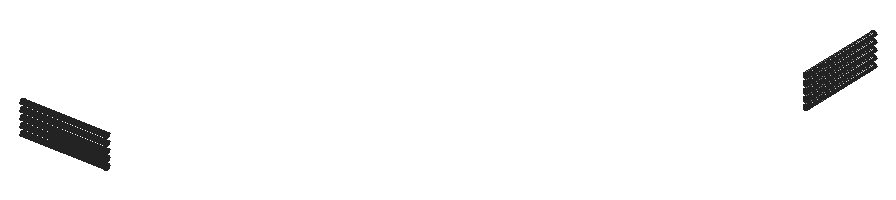
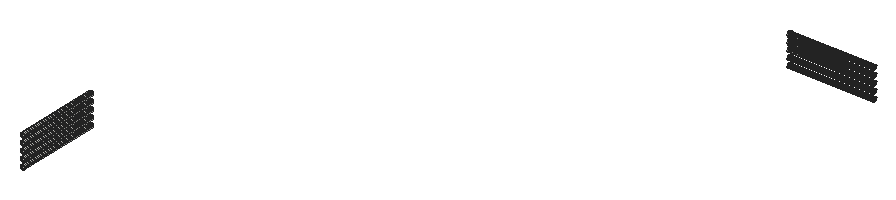
# SketchUp Ruby script. Lengths in inches.
U = 1.inch
M = Sketchup.active_model
def pt(a) = Geom::Point3d.new(a.map { |v| v * U })
def face(e, loops, mat)
  f = e.add_face(loops[0].map { |a| pt(a) })
  loops[1..].each { |l| e.add_face(l.map { |a| pt(a) }).erase! }
  f.material = f.back_material = mat if mat
  f
end
# faces: each face lists its corners as indices into pts; further lists are holes
def faces(e, pts, list, mat = nil) = list.each { |f| face(e, (f[0].is_a?(Array) ? f : [f]).map { |l| l.map { |i| pts[i] } }, mat) }
# xy, xz, yz: faces in a plane at the given z, y or x. An outline is a flat list of corners, or four numbers for a rectangle; further outlines are holes
def ring(l) = l.size == 4 ? [[l[0], l[1]], [l[2], l[1]], [l[2], l[3]], [l[0], l[3]]] : l.each_slice(2).to_a
def flat(e, list, mat, &to3) = list.each { |f| face(e, (f[0].is_a?(Array) ? f : [f]).map { |l| ring(l).map { |u, v| to3.(u, v) } }, mat) }
def xy(e, z, list, mat = nil) = flat(e, list, mat) { |x, y| [x, y, z] }
def xz(e, y, list, mat = nil) = flat(e, list, mat) { |x, z| [x, y, z] }
def yz(e, x, list, mat = nil) = flat(e, list, mat) { |y, z| [x, y, z] }
def lines(e, pts, list) = list.each { |a, b| e.add_line(pt(pts[a]), pt(pts[b])) }
# prism: a flat outline (further loops are holes) pulled along v
def prism(e, loops, v, mat = nil)
  f = face(e, loops, mat); d = Geom::Vector3d.new(v.map { |x| x * U })
  f.pushpull(f.normal.samedirection?(d) ? d.length : -d.length)
end
def box(e, o, s, mat = nil) = prism(e, [[o, [o[0] + s[0], o[1], o[2]], [o[0] + s[0], o[1] + s[1], o[2]], [o[0], o[1] + s[1], o[2]]]], [0, 0, s[2]], mat)
def at(x, y, z, deg = 0) = Geom::Transformation.translation(pt([x, y, z])) * Geom::Transformation.rotation(ORIGIN, Z_AXIS, deg.degrees)
def axes(o, x, y, z) = Geom::Transformation.new([*x, 0, *y, 0, *z, 0, *pt(o).to_a, 1])
def part(name) = M.definitions.add(name)
# library, detail: a bought-in or finely detailed component or shape, given as its bounding box
def library(name, o, s) = part(name).tap { |d| box(d.entities, o, s) }
def detail(e, o, s) = box(e.add_group.entities, o, s)
def put(e, d, t, mat = nil) = e.add_instance(d, t).tap { |i| i.material = mat if mat }
def group(e, t, mat = nil) = e.add_group.tap { |g| g.transformation = t; g.material = mat if mat }.entities
root = M.entities
p = [[922.01,48.34,1317.02],[922.01,47.38,1317.14],[778.64,47.38,1317.14],[778.64,48.34,1317.02],[922.01,49.29,1317.14],[778.64,49.29,1317.14],
  [1535.52,886.83,1317.14],[1536.47,886.83,1317.02],[1536.47,743.45,1317.02],[1535.52,743.45,1317.14],[1537.43,886.83,1317.14],[1537.43,743.45,1317.14],
  [922.01,46.5,1317.51],[778.64,46.5,1317.51],[922.01,50.18,1317.51],[778.64,50.18,1317.51],[1534.63,886.83,1317.51],[1534.63,743.45,1317.51],
  [1538.32,886.83,1317.51],[1538.32,743.45,1317.51],[922.01,45.73,1318.1],[778.64,45.73,1318.1],[922.01,50.95,1318.1],[778.64,50.95,1318.1],
  [1533.87,886.83,1318.1],[1533.87,743.45,1318.1],[1539.08,886.83,1318.1],[1539.08,743.45,1318.1],[922.01,45.15,1318.86],[778.64,45.15,1318.86],
  [922.01,51.53,1318.86],[778.64,51.53,1318.86],[1533.28,886.83,1318.86],[1533.28,743.45,1318.86],[1539.67,886.83,1318.86],[1539.67,743.45,1318.86],
  [922.01,44.78,1319.75],[778.64,44.78,1319.75],[922.01,51.9,1319.75],[778.64,51.9,1319.75],[1532.91,886.83,1319.75],[1532.91,743.45,1319.75],
  [1540.03,886.83,1319.75],[1540.03,743.45,1319.75],[922.01,44.65,1320.7],[778.64,44.65,1320.7],[922.01,52.03,1320.7],[778.64,52.03,1320.7],
  [1532.79,886.83,1320.7],[1532.79,743.45,1320.7],[1540.16,886.83,1320.7],[1540.16,743.45,1320.7],[922.01,44.78,1321.66],[778.64,44.78,1321.66],
  [922.01,51.9,1321.66],[778.64,51.9,1321.66],[1532.91,886.83,1321.66],[1532.91,743.45,1321.66],[1540.03,886.83,1321.66],[1540.03,743.45,1321.66],
  [922.01,45.15,1322.55],[778.64,45.15,1322.55],[922.01,51.53,1322.55],[778.64,51.53,1322.55],[1533.28,886.83,1322.55],[1533.28,743.45,1322.55],
  [1539.67,886.83,1322.55],[1539.67,743.45,1322.55],[922.01,45.73,1323.3125],[778.64,45.73,1323.3125],[922.01,50.95,1323.3125],[778.64,50.95,1323.3125],
  [1533.87,886.83,1323.3125],[1533.87,743.45,1323.3125],[1539.08,886.83,1323.3125],[1539.08,743.45,1323.3125],[922.01,46.5,1323.9],[778.64,46.5,1323.9],
  [922.01,50.18,1323.9],[778.64,50.18,1323.9],[1534.63,886.83,1323.9],[1534.63,743.45,1323.9],[1538.32,886.83,1323.9],[1538.32,743.45,1323.9],
  [922.01,47.38,1324.27],[778.64,47.38,1324.27],[922.01,49.29,1324.27],[778.64,49.29,1324.27],[1535.52,886.83,1324.27],[1535.52,743.45,1324.27],
  [1537.43,886.83,1324.27],[1537.43,743.45,1324.27],[922.01,48.34,1324.39],[778.64,48.34,1324.39],[1536.47,886.83,1324.39],[1536.47,743.45,1324.39],
  [922.01,48.34,1329.02],[922.01,47.38,1329.14],[778.64,47.38,1329.14],[778.64,48.34,1329.02],[922.01,49.29,1329.14],[778.64,49.29,1329.14],
  [1535.52,886.83,1329.14],[1536.47,886.83,1329.02],[1536.47,743.45,1329.02],[1535.52,743.45,1329.14],[1537.43,886.83,1329.14],[1537.43,743.45,1329.14],
  [922.01,46.5,1329.51],[778.64,46.5,1329.51],[922.01,50.18,1329.51],[778.64,50.18,1329.51],[1534.63,886.83,1329.51],[1534.63,743.45,1329.51],
  [1538.32,886.83,1329.51],[1538.32,743.45,1329.51],[922.01,45.73,1330.1],[778.64,45.73,1330.1],[922.01,50.95,1330.1],[778.64,50.95,1330.1],
  [1533.87,886.83,1330.1],[1533.87,743.45,1330.1],[1539.08,886.83,1330.1],[1539.08,743.45,1330.1],[922.01,45.15,1330.86],[778.64,45.15,1330.86],
  [922.01,51.53,1330.86],[778.64,51.53,1330.86],[1533.28,886.83,1330.86],[1533.28,743.45,1330.86],[1539.67,886.83,1330.86],[1539.67,743.45,1330.86],
  [922.01,44.78,1331.75],[778.64,44.78,1331.75],[922.01,51.9,1331.75],[778.64,51.9,1331.75],[1532.91,886.83,1331.75],[1532.91,743.45,1331.75],
  [1540.03,886.83,1331.75],[1540.03,743.45,1331.75],[922.01,44.65,1332.7],[778.64,44.65,1332.7],[922.01,52.03,1332.7],[778.64,52.03,1332.7],
  [1532.79,886.83,1332.7],[1532.79,743.45,1332.7],[1540.16,886.83,1332.7],[1540.16,743.45,1332.7],[922.01,44.78,1333.66],[778.64,44.78,1333.66],
  [922.01,51.9,1333.66],[778.64,51.9,1333.66],[1532.91,886.83,1333.66],[1532.91,743.45,1333.66],[1540.03,886.83,1333.66],[1540.03,743.45,1333.66],
  [922.01,45.15,1334.55],[778.64,45.15,1334.55],[922.01,51.53,1334.55],[778.64,51.53,1334.55],[1533.28,886.83,1334.55],[1533.28,743.45,1334.55],
  [1539.67,886.83,1334.55],[1539.67,743.45,1334.55],[922.01,45.73,1335.3125],[778.64,45.73,1335.3125],[922.01,50.95,1335.3125],[778.64,50.95,1335.3125],
  [1533.87,886.83,1335.3125],[1533.87,743.45,1335.3125],[1539.08,886.83,1335.3125],[1539.08,743.45,1335.3125],[922.01,46.5,1335.9],[778.64,46.5,1335.9],
  [922.01,50.18,1335.9],[778.64,50.18,1335.9],[1534.63,886.83,1335.9],[1534.63,743.45,1335.9],[1538.32,886.83,1335.9],[1538.32,743.45,1335.9],
  [922.01,47.38,1336.27],[778.64,47.38,1336.27],[922.01,49.29,1336.27],[778.64,49.29,1336.27],[1535.52,886.83,1336.27],[1535.52,743.45,1336.27],
  [1537.43,886.83,1336.27],[1537.43,743.45,1336.27],[922.01,48.34,1336.39],[778.64,48.34,1336.39],[1536.47,886.83,1336.39],[1536.47,743.45,1336.39],
  [922.01,48.34,1341.02],[922.01,47.38,1341.14],[778.64,47.38,1341.14],[778.64,48.34,1341.02],[922.01,49.29,1341.14],[778.64,49.29,1341.14],
  [1535.52,886.83,1341.14],[1536.47,886.83,1341.02],[1536.47,743.45,1341.02],[1535.52,743.45,1341.14],[1537.43,886.83,1341.14],[1537.43,743.45,1341.14],
  [922.01,46.5,1341.51],[778.64,46.5,1341.51],[922.01,50.18,1341.51],[778.64,50.18,1341.51],[1534.63,886.83,1341.51],[1534.63,743.45,1341.51],
  [1538.32,886.83,1341.51],[1538.32,743.45,1341.51],[922.01,45.73,1342.1],[778.64,45.73,1342.1],[922.01,50.95,1342.1],[778.64,50.95,1342.1],
  [1533.87,886.83,1342.1],[1533.87,743.45,1342.1],[1539.08,886.83,1342.1],[1539.08,743.45,1342.1],[922.01,45.15,1342.86],[778.64,45.15,1342.86],
  [922.01,51.53,1342.86],[778.64,51.53,1342.86],[1533.28,886.83,1342.86],[1533.28,743.45,1342.86],[1539.67,886.83,1342.86],[1539.67,743.45,1342.86],
  [922.01,44.78,1343.75],[778.64,44.78,1343.75],[922.01,51.9,1343.75],[778.64,51.9,1343.75],[1532.91,886.83,1343.75],[1532.91,743.45,1343.75],
  [1540.03,886.83,1343.75],[1540.03,743.45,1343.75],[922.01,44.65,1344.7],[778.64,44.65,1344.7],[922.01,52.03,1344.7],[778.64,52.03,1344.7],
  [1532.79,886.83,1344.7],[1532.79,743.45,1344.7],[1540.16,886.83,1344.7],[1540.16,743.45,1344.7],[922.01,44.78,1345.66],[778.64,44.78,1345.66],
  [922.01,51.9,1345.66],[778.64,51.9,1345.66],[1532.91,886.83,1345.66],[1532.91,743.45,1345.66],[1540.03,886.83,1345.66],[1540.03,743.45,1345.66],
  [922.01,45.15,1346.55],[778.64,45.15,1346.55],[922.01,51.53,1346.55],[778.64,51.53,1346.55],[1533.28,886.83,1346.55],[1533.28,743.45,1346.55],
  [1539.67,886.83,1346.55],[1539.67,743.45,1346.55],[922.01,45.73,1347.3125],[778.64,45.73,1347.3125],[922.01,50.95,1347.3125],[778.64,50.95,1347.3125],
  [1533.87,886.83,1347.3125],[1533.87,743.45,1347.3125],[1539.08,886.83,1347.3125],[1539.08,743.45,1347.3125],[922.01,46.5,1347.9],[778.64,46.5,1347.9],
  [922.01,50.18,1347.9],[778.64,50.18,1347.9],[1534.63,886.83,1347.9],[1534.63,743.45,1347.9],[1538.32,886.83,1347.9],[1538.32,743.45,1347.9],
  [922.01,47.38,1348.27],[778.64,47.38,1348.27],[922.01,49.29,1348.27],[778.64,49.29,1348.27],[1535.52,886.83,1348.27],[1535.52,743.45,1348.27],
  [1537.43,886.83,1348.27],[1537.43,743.45,1348.27],[922.01,48.34,1348.39],[778.64,48.34,1348.39],[1536.47,886.83,1348.39],[1536.47,743.45,1348.39],
  [922.01,48.34,1353.02],[922.01,47.38,1353.14],[778.64,47.38,1353.14],[778.64,48.34,1353.02],[922.01,49.29,1353.14],[778.64,49.29,1353.14],
  [1535.52,886.83,1353.14],[1536.47,886.83,1353.02],[1536.47,743.45,1353.02],[1535.52,743.45,1353.14],[1537.43,886.83,1353.14],[1537.43,743.45,1353.14],
  [922.01,46.5,1353.51],[778.64,46.5,1353.51],[922.01,50.18,1353.51],[778.64,50.18,1353.51],[1534.63,886.83,1353.51],[1534.63,743.45,1353.51],
  [1538.32,886.83,1353.51],[1538.32,743.45,1353.51],[922.01,45.73,1354.1],[778.64,45.73,1354.1],[922.01,50.95,1354.1],[778.64,50.95,1354.1],
  [1533.87,886.83,1354.1],[1533.87,743.45,1354.1],[1539.08,886.83,1354.1],[1539.08,743.45,1354.1],[922.01,45.15,1354.86],[778.64,45.15,1354.86],
  [922.01,51.53,1354.86],[778.64,51.53,1354.86],[1533.28,886.83,1354.86],[1533.28,743.45,1354.86],[1539.67,886.83,1354.86],[1539.67,743.45,1354.86],
  [922.01,44.78,1355.75],[778.64,44.78,1355.75],[922.01,51.9,1355.75],[778.64,51.9,1355.75],[1532.91,886.83,1355.75],[1532.91,743.45,1355.75],
  [1540.03,886.83,1355.75],[1540.03,743.45,1355.75],[922.01,44.65,1356.7],[778.64,44.65,1356.7],[922.01,52.03,1356.7],[778.64,52.03,1356.7],
  [1532.79,886.83,1356.7],[1532.79,743.45,1356.7],[1540.16,886.83,1356.7],[1540.16,743.45,1356.7],[922.01,44.78,1357.66],[778.64,44.78,1357.66],
  [922.01,51.9,1357.66],[778.64,51.9,1357.66],[1532.91,886.83,1357.66],[1532.91,743.45,1357.66],[1540.03,886.83,1357.66],[1540.03,743.45,1357.66],
  [922.01,45.15,1358.55],[778.64,45.15,1358.55],[922.01,51.53,1358.55],[778.64,51.53,1358.55],[1533.28,886.83,1358.55],[1533.28,743.45,1358.55],
  [1539.67,886.83,1358.55],[1539.67,743.45,1358.55],[922.01,45.73,1359.3125],[778.64,45.73,1359.3125],[922.01,50.95,1359.3125],[778.64,50.95,1359.3125],
  [1533.87,886.83,1359.3125],[1533.87,743.45,1359.3125],[1539.08,886.83,1359.3125],[1539.08,743.45,1359.3125],[922.01,46.5,1359.9],[778.64,46.5,1359.9],
  [922.01,50.18,1359.9],[778.64,50.18,1359.9],[1534.63,886.83,1359.9],[1534.63,743.45,1359.9],[1538.32,886.83,1359.9],[1538.32,743.45,1359.9],
  [922.01,47.38,1360.27],[778.64,47.38,1360.27],[922.01,49.29,1360.27],[778.64,49.29,1360.27],[1535.52,886.83,1360.27],[1535.52,743.45,1360.27],
  [1537.43,886.83,1360.27],[1537.43,743.45,1360.27],[922.01,48.34,1360.39],[778.64,48.34,1360.39],[1536.47,886.83,1360.39],[1536.47,743.45,1360.39],
  [922.01,48.34,1365.02],[922.01,47.38,1365.14],[778.64,47.38,1365.14],[778.64,48.34,1365.02],[922.01,49.29,1365.14],[778.64,49.29,1365.14],
  [1535.52,886.83,1365.14],[1536.47,886.83,1365.02],[1536.47,743.45,1365.02],[1535.52,743.45,1365.14],[1537.43,886.83,1365.14],[1537.43,743.45,1365.14],
  [922.01,46.5,1365.51],[778.64,46.5,1365.51],[922.01,50.18,1365.51],[778.64,50.18,1365.51],[1534.63,886.83,1365.51],[1534.63,743.45,1365.51],
  [1538.32,886.83,1365.51],[1538.32,743.45,1365.51],[922.01,45.73,1366.1],[778.64,45.73,1366.1],[922.01,50.95,1366.1],[778.64,50.95,1366.1],
  [1533.87,886.83,1366.1],[1533.87,743.45,1366.1],[1539.08,886.83,1366.1],[1539.08,743.45,1366.1],[922.01,45.15,1366.86],[778.64,45.15,1366.86],
  [922.01,51.53,1366.86],[778.64,51.53,1366.86],[1533.28,886.83,1366.86],[1533.28,743.45,1366.86],[1539.67,886.83,1366.86],[1539.67,743.45,1366.86],
  [922.01,44.78,1367.75],[778.64,44.78,1367.75],[922.01,51.9,1367.75],[778.64,51.9,1367.75],[1532.91,886.83,1367.75],[1532.91,743.45,1367.75],
  [1540.03,886.83,1367.75],[1540.03,743.45,1367.75],[922.01,44.65,1368.7],[778.64,44.65,1368.7],[922.01,52.03,1368.7],[778.64,52.03,1368.7],
  [1532.79,886.83,1368.7],[1532.79,743.45,1368.7],[1540.16,886.83,1368.7],[1540.16,743.45,1368.7],[922.01,44.78,1369.66],[778.64,44.78,1369.66],
  [922.01,51.9,1369.66],[778.64,51.9,1369.66],[1532.91,886.83,1369.66],[1532.91,743.45,1369.66],[1540.03,886.83,1369.66],[1540.03,743.45,1369.66],
  [922.01,45.15,1370.55],[778.64,45.15,1370.55],[922.01,51.53,1370.55],[778.64,51.53,1370.55],[1533.28,886.83,1370.55],[1533.28,743.45,1370.55],
  [1539.67,886.83,1370.55],[1539.67,743.45,1370.55],[922.01,45.73,1371.3125],[778.64,45.73,1371.3125],[922.01,50.95,1371.3125],[778.64,50.95,1371.3125],
  [1533.87,886.83,1371.3125],[1533.87,743.45,1371.3125],[1539.08,886.83,1371.3125],[1539.08,743.45,1371.3125],[922.01,46.5,1371.9],[778.64,46.5,1371.9],
  [922.01,50.18,1371.9],[778.64,50.18,1371.9],[1534.63,886.83,1371.9],[1534.63,743.45,1371.9],[1538.32,886.83,1371.9],[1538.32,743.45,1371.9],
  [922.01,47.38,1372.27],[778.64,47.38,1372.27],[922.01,49.29,1372.27],[778.64,49.29,1372.27],[1535.52,886.83,1372.27],[1535.52,743.45,1372.27],
  [1537.43,886.83,1372.27],[1537.43,743.45,1372.27],[922.01,48.34,1372.39],[778.64,48.34,1372.39],[1536.47,886.83,1372.39],[1536.47,743.45,1372.39]]
faces(root,p,[[0,1,2,3],[4,0,3,5],[6,7,8,9],[7,10,11,8],[1,12,13,2],[14,4,5,15],[16,6,9,17],[10,18,19,11],
  [12,20,21,13],[22,14,15,23],[24,16,17,25],[18,26,27,19],[20,28,29,21],[30,22,23,31],[32,24,25,33],[26,34,35,27],
  [28,36,37,29],[38,30,31,39],[40,32,33,41],[34,42,43,35],[36,44,45,37],[46,38,39,47],[48,40,41,49],[42,50,51,43],
  [44,52,53,45],[54,46,47,55],[56,48,49,57],[50,58,59,51],[52,60,61,53],[62,54,55,63],[64,56,57,65],[58,66,67,59],
  [60,68,69,61],[70,62,63,71],[72,64,65,73],[66,74,75,67],[68,76,77,69],[78,70,71,79],[80,72,73,81],[74,82,83,75],
  [76,84,85,77],[86,78,79,87],[88,80,81,89],[82,90,91,83],[84,92,93,85],[92,86,87,93],[94,88,89,95],[90,94,95,91],
  [96,97,98,99],[100,96,99,101],[102,103,104,105],[103,106,107,104],[97,108,109,98],[110,100,101,111],[112,102,105,113],[106,114,115,107],
  [108,116,117,109],[118,110,111,119],[120,112,113,121],[114,122,123,115],[116,124,125,117],[126,118,119,127],[128,120,121,129],[122,130,131,123],
  [124,132,133,125],[134,126,127,135],[136,128,129,137],[130,138,139,131],[132,140,141,133],[142,134,135,143],[144,136,137,145],[138,146,147,139],
  [140,148,149,141],[150,142,143,151],[152,144,145,153],[146,154,155,147],[148,156,157,149],[158,150,151,159],[160,152,153,161],[154,162,163,155],
  [156,164,165,157],[166,158,159,167],[168,160,161,169],[162,170,171,163],[164,172,173,165],[174,166,167,175],[176,168,169,177],[170,178,179,171],
  [172,180,181,173],[182,174,175,183],[184,176,177,185],[178,186,187,179],[180,188,189,181],[188,182,183,189],[190,184,185,191],[186,190,191,187],
  [192,193,194,195],[196,192,195,197],[198,199,200,201],[199,202,203,200],[193,204,205,194],[206,196,197,207],[208,198,201,209],[202,210,211,203],
  [204,212,213,205],[214,206,207,215],[216,208,209,217],[210,218,219,211],[212,220,221,213],[222,214,215,223],[224,216,217,225],[218,226,227,219],
  [220,228,229,221],[230,222,223,231],[232,224,225,233],[226,234,235,227],[228,236,237,229],[238,230,231,239],[240,232,233,241],[234,242,243,235],
  [236,244,245,237],[246,238,239,247],[248,240,241,249],[242,250,251,243],[244,252,253,245],[254,246,247,255],[256,248,249,257],[250,258,259,251],
  [252,260,261,253],[262,254,255,263],[264,256,257,265],[258,266,267,259],[260,268,269,261],[270,262,263,271],[272,264,265,273],[266,274,275,267],
  [268,276,277,269],[278,270,271,279],[280,272,273,281],[274,282,283,275],[276,284,285,277],[284,278,279,285],[286,280,281,287],[282,286,287,283],
  [288,289,290,291],[292,288,291,293],[294,295,296,297],[295,298,299,296],[289,300,301,290],[302,292,293,303],[304,294,297,305],[298,306,307,299],
  [300,308,309,301],[310,302,303,311],[312,304,305,313],[306,314,315,307],[308,316,317,309],[318,310,311,319],[320,312,313,321],[314,322,323,315],
  [316,324,325,317],[326,318,319,327],[328,320,321,329],[322,330,331,323],[324,332,333,325],[334,326,327,335],[336,328,329,337],[330,338,339,331],
  [332,340,341,333],[342,334,335,343],[344,336,337,345],[338,346,347,339],[340,348,349,341],[350,342,343,351],[352,344,345,353],[346,354,355,347],
  [348,356,357,349],[358,350,351,359],[360,352,353,361],[354,362,363,355],[356,364,365,357],[366,358,359,367],[368,360,361,369],[362,370,371,363],
  [364,372,373,365],[374,366,367,375],[376,368,369,377],[370,378,379,371],[372,380,381,373],[380,374,375,381],[382,376,377,383],[378,382,383,379],
  [384,385,386,387],[388,384,387,389],[390,391,392,393],[391,394,395,392],[385,396,397,386],[398,388,389,399],[400,390,393,401],[394,402,403,395],
  [396,404,405,397],[406,398,399,407],[408,400,401,409],[402,410,411,403],[404,412,413,405],[414,406,407,415],[416,408,409,417],[410,418,419,411],
  [412,420,421,413],[422,414,415,423],[424,416,417,425],[418,426,427,419],[420,428,429,421],[430,422,423,431],[432,424,425,433],[426,434,435,427],
  [428,436,437,429],[438,430,431,439],[440,432,433,441],[434,442,443,435],[436,444,445,437],[446,438,439,447],[448,440,441,449],[442,450,451,443],
  [444,452,453,445],[454,446,447,455],[456,448,449,457],[450,458,459,451],[452,460,461,453],[462,454,455,463],[464,456,457,465],[458,466,467,459],
  [460,468,469,461],[470,462,463,471],[472,464,465,473],[466,474,475,467],[468,476,477,469],[476,470,471,477],[478,472,473,479],[474,478,479,475]])
